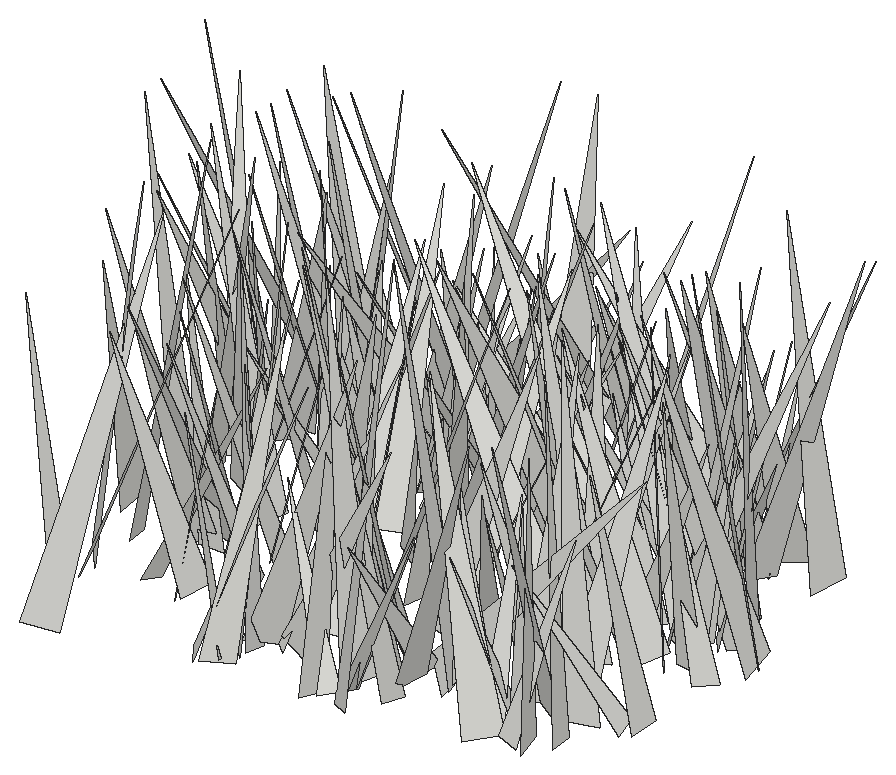
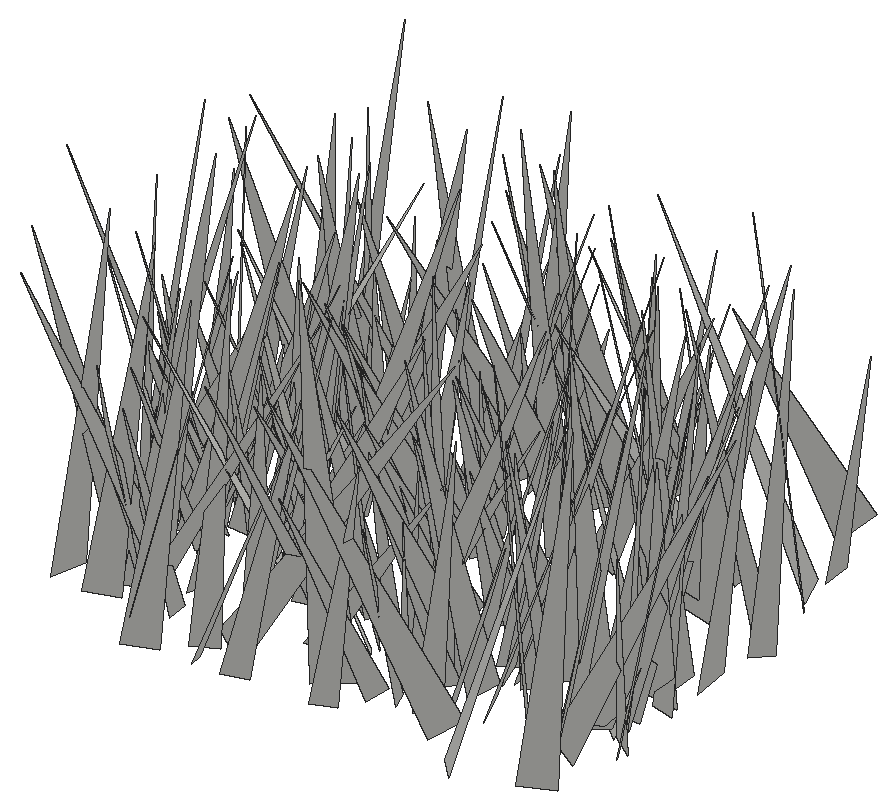
# SketchUp Ruby script. Lengths in inches.
U = 1.inch
M = Sketchup.active_model
def pt(a) = Geom::Point3d.new(a.map { |v| v * U })
def face(e, loops, mat)
  f = e.add_face(loops[0].map { |a| pt(a) })
  loops[1..].each { |l| e.add_face(l.map { |a| pt(a) }).erase! }
  f.material = f.back_material = mat if mat
  f
end
# faces: each face lists its corners as indices into pts; further lists are holes
def faces(e, pts, list, mat = nil) = list.each { |f| face(e, (f[0].is_a?(Array) ? f : [f]).map { |l| l.map { |i| pts[i] } }, mat) }
# xy, xz, yz: faces in a plane at the given z, y or x. An outline is a flat list of corners, or four numbers for a rectangle; further outlines are holes
def ring(l) = l.size == 4 ? [[l[0], l[1]], [l[2], l[1]], [l[2], l[3]], [l[0], l[3]]] : l.each_slice(2).to_a
def flat(e, list, mat, &to3) = list.each { |f| face(e, (f[0].is_a?(Array) ? f : [f]).map { |l| ring(l).map { |u, v| to3.(u, v) } }, mat) }
def xy(e, z, list, mat = nil) = flat(e, list, mat) { |x, y| [x, y, z] }
def xz(e, y, list, mat = nil) = flat(e, list, mat) { |x, z| [x, y, z] }
def yz(e, x, list, mat = nil) = flat(e, list, mat) { |y, z| [x, y, z] }
def lines(e, pts, list) = list.each { |a, b| e.add_line(pt(pts[a]), pt(pts[b])) }
# prism: a flat outline (further loops are holes) pulled along v
def prism(e, loops, v, mat = nil)
  f = face(e, loops, mat); d = Geom::Vector3d.new(v.map { |x| x * U })
  f.pushpull(f.normal.samedirection?(d) ? d.length : -d.length)
end
def box(e, o, s, mat = nil) = prism(e, [[o, [o[0] + s[0], o[1], o[2]], [o[0] + s[0], o[1] + s[1], o[2]], [o[0], o[1] + s[1], o[2]]]], [0, 0, s[2]], mat)
def at(x, y, z, deg = 0) = Geom::Transformation.translation(pt([x, y, z])) * Geom::Transformation.rotation(ORIGIN, Z_AXIS, deg.degrees)
def axes(o, x, y, z) = Geom::Transformation.new([*x, 0, *y, 0, *z, 0, *pt(o).to_a, 1])
def part(name) = M.definitions.add(name)
# library, detail: a bought-in or finely detailed component or shape, given as its bounding box
def library(name, o, s) = part(name).tap { |d| box(d.entities, o, s) }
def detail(e, o, s) = box(e.add_group.entities, o, s)
def put(e, d, t, mat = nil) = e.add_instance(d, t).tap { |i| i.material = mat if mat }
def group(e, t, mat = nil) = e.add_group.tap { |g| g.transformation = t; g.material = mat if mat }.entities
root = M.entities
c1 = part("fur_instance\#9")
p = [[0.8125,0,1.79],[0.67,-0.02,1.48],[0,-0.11,0],[0,0.11,0]]
faces(c1.entities,p,[[0,1,2,3]])
put(root,c1,axes([79.35,396.46,-27.1],[3.86855,-0.79855,0.19754],[-0.81455,-3.85123,0.38332],[-0.11496,0.41562,3.93147]))
put(root,c1,axes([73.47,395.12,-27.1],[4.56753,3.50086,0.36537],[3.49009,-4.58212,0.27435],[-0.45689,-0.00383,5.74831]))
put(root,c1,axes([78.98,395.87,-27.1],[-2.26305,3.25436,0.20739],[3.19812,2.16563,0.91504],[-0.63708,-0.68879,3.8568]))
put(root,c1,axes([74.48,395.55,-27.1],[-4.28089,-1.18354,0.47624],[-1.27514,3.91753,-1.72642],[-0.03977,1.79046,4.09221]))
put(root,c1,axes([86.23,399.45,-27.1],[-2.59583,-7.17613,0.91864],[-6.91744,2.74775,1.9178],[2.11891,0.17907,7.38629]))
put(root,c1,axes([66.48,396.31,-27.1],[-5.31115,0.249,1.00047],[0.14264,5.37711,-0.58108],[1.02108,0.54405,5.28514]))
put(root,c1,axes([76,397.62,-27.1],[0.54416,-5.67013,1.84078],[-5.27926,0.40028,2.79359],[2.76917,1.87733,4.9641]))
put(root,c1,axes([80.71,398.32,-27.1],[6.6655,-1.52718,0.22941],[-1.49066,-6.62814,-0.81212],[-0.40351,-0.74118,6.78982]))
put(root,c1,axes([80.7,399.42,-27.1],[3.27584,-2.78093,0.2499],[-2.38988,-2.99185,-1.96583],[-1.44378,-1.35736,3.82103]))
put(root,c1,axes([86.86,397.32,-27.1],[5.38301,1.51294,2.42188],[1.75431,-5.82988,-0.25732],[-2.2532,-0.92457,5.58566]))
put(root,c1,axes([74.49,395.2,-27.1],[-4.85985,3.92503,1.53679],[3.59209,5.08366,-1.6245],[2.20555,0.36911,6.032]))
put(root,c1,axes([85.26,396.76,-27.1],[-5.2406,4.407,1.34408],[4.57378,5.22157,0.71269],[0.55566,-1.41624,6.81011]))
put(root,c1,axes([78.59,395.48,-27.1],[-7.01527,0.64484,2.20419],[0.06996,7.14138,-1.86657],[2.29551,1.75305,6.79307]))
put(root,c1,axes([68.03,393.23,-27.1],[-6.65412,4.03174,0.74119],[3.28122,6.08544,-3.64454],[2.45722,2.79179,6.87384]))
put(root,c1,axes([74.87,397.32,-27.1],[5.22316,-4.20753,1.34718],[-4.41725,-5.01042,1.47756],[-0.07792,1.998,6.54228]))
put(root,c1,axes([79.34,397.22,-27.1],[-7.46216,1.5868,2.36089],[1.65538,7.81249,-0.01867],[2.31332,-0.47194,7.62898]))
put(root,c1,axes([70.68,398.75,-27.1],[-5.0365,1.95588,2.0654],[2.56555,4.93734,1.5806],[1.22852,-2.29236,5.16658]))
put(root,c1,axes([85.71,398.26,-27.1],[-3.47043,-1.20582,0.35373],[-1.16309,3.47557,0.43669],[0.47575,-0.29913,3.64791]))
put(root,c1,axes([70.1,398.38,-27.1],[4.41125,2.39111,1.26664],[2.67652,-4.21168,-1.37073],[-0.39751,-1.82353,4.82677]))
put(root,c1,axes([86.12,397.06,-27.1],[1.17442,4.10835,0.87727],[4.16659,-1.02282,-0.78793],[0.5364,-1.0501,4.19964]))
put(root,c1,axes([79.95,395.3,-27.1],[4.59054,6.55576,1.84003],[6.00661,-4.94402,2.62946],[-3.20693,0.124,7.5589]))
put(root,c1,axes([79.47,399.59,-27.1],[-3.91198,-5.41617,1.52932],[-5.50053,4.07361,0.35664],[1.19076,1.02376,6.67167]))
put(root,c1,axes([74.93,396.75,-27.1],[-6.75602,-0.97126,1.58692],[-1.43223,6.52998,-2.10085],[1.1876,2.34979,6.49412]))
put(root,c1,axes([85.06,397.44,-27.1],[-1.60634,4.05647,0.77587],[4.09581,1.67158,-0.25963],[0.53033,-0.623,4.35521]))
put(root,c1,axes([74.64,396.21,-27.1],[5.18637,5.57386,2.23152],[5.04396,-5.64447,2.37581],[-3.2567,0.13438,7.23339]))
put(root,c1,axes([81.04,396.94,-27.1],[-7.866,-1.33504,0.19154],[-1.32695,7.45779,-2.51268],[-0.24134,2.50839,7.5725]))
put(root,c1,axes([83.48,398.91,-27.1],[-3.08367,2.72536,1.78242],[3.08151,3.23588,0.38343],[1.05304,-1.48834,4.09751]))
put(root,c1,axes([72.75,399.54,-27.1],[-2.53313,-4.37285,1.78451],[-4.47538,2.86942,0.67851],[1.50904,1.16947,5.00781]))
put(root,c1,axes([66.24,398.49,-27.1],[5.70767,4.90783,2.44546],[5.23724,-5.92496,-0.33273],[-1.62433,-1.85811,7.52021]))
put(root,c1,axes([66.44,397.78,-27.1],[7.55875,3.30018,0.58934],[3.3113,-7.57673,-0.04195],[-0.52327,-0.27436,8.24768]))
put(root,c1,axes([81.13,399.31,-27.1],[5.03462,6.0848,0.40692],[5.07887,-3.8915,-4.64748],[3.37572,-3.22012,6.38538]))
put(root,c1,axes([85.7,398.17,-27.1],[-3.90689,0.46662,1.17538],[0.26281,4.03296,-0.72751],[1.23701,0.61693,3.86682]))
put(root,c1,axes([88.72,400.48,-27.1],[-4.09373,-0.36711,0.23804],[-0.24891,3.79616,1.57392],[0.35983,-1.55061,3.79686]))
put(root,c1,axes([75.23,397.73,-27.1],[3.93505,4.96293,0.50565],[4.97977,-3.8695,-0.7745],[0.29702,-0.87596,6.28613]))
put(root,c1,axes([72.21,400.37,-27.1],[-5.06877,-1.96642,0.89661],[-1.81084,5.11214,0.97466],[1.17965,-0.60192,5.34876]))
put(root,c1,axes([87.65,398.17,-27.1],[-6.31895,-1.30533,1.91515],[-1.71826,6.37081,-1.32708],[1.5554,1.73484,6.31441]))
put(root,c1,axes([81.94,399.49,-27.1],[-7.67624,-2.38765,2.18106],[-2.53698,7.93,-0.24775],[2.0054,0.89261,8.03519]))
put(root,c1,axes([70.76,401.5,-27.1],[-3.28751,-5.48957,1.02333],[-5.33666,3.43821,1.29963],[1.64396,0.18343,6.2653]))
put(root,c1,axes([68.89,398.44,-27.1],[4.92318,-0.35306,0.35659],[-0.43613,-4.74982,1.31852],[-0.24819,1.34315,4.75646]))
put(root,c1,axes([78.87,397.71,-27.1],[-4.6642,0.46344,0.8289],[0.1067,4.38406,-1.85075],[0.94364,1.79496,4.30631]))
put(root,c1,axes([69.5625,402.18,-27.1],[-1.29873,-6.18935,0.13887],[-6.18983,1.30082,0.08883],[0.11547,0.11765,6.32352]))
put(root,c1,axes([74.83,401.34,-27.1],[0.15208,-7.64456,1.76209],[-7.47072,0.39677,2.36609],[2.3943,1.72356,7.27077]))
put(root,c1,axes([84.03,400.91,-27.1],[-0.63245,-3.70623,0.66325],[-3.76509,0.62047,-0.12308],[-0.01169,0.67448,3.75779]))
put(root,c1,axes([89.28,400.84,-27.1],[-5.12264,0.34016,1.65759],[0.60899,5.30124,0.79415],[1.57874,-0.94118,5.07212]))
put(root,c1,axes([79.77,398.69,-27.1],[-7.1733,-2.93015,0.73361],[-2.97558,6.52972,-3.01478],[-0.51951,3.05896,7.13815]))
put(root,c1,axes([68.76,401.6,-27.1],[-0.74223,-7.02206,1.66779],[-7.14663,0.48084,-1.156],[-1.00829,1.76103,6.96591]))
put(root,c1,axes([77.93,401.3125,-27.1],[-1.24841,-4.57565,0.91997],[-4.66472,1.19209,-0.401],[-0.15278,0.99186,4.72592]))
put(root,c1,axes([80.73,402.82,-27.1],[5.43533,-0.93824,0.08866],[-0.80913,-4.91198,-2.3767],[-0.48317,-2.32876,4.97739]))
put(root,c1,axes([64.89,402.51,-27.1],[6.40589,-1.32849,1.4611],[-0.83624,-6.31798,-2.07823],[-1.78897,-1.80373,6.20333]))
put(root,c1,axes([87.33,399.73,-27.1],[-0.74799,6.94474,2.29097],[7.27165,0.46217,0.97314],[-0.77532,-2.36525,6.91678]))
put(root,c1,axes([73.6,400.71,-27.1],[-0.2537,5.53184,2.90433],[5.7111,-0.97344,2.35297],[-2.53371,-2.74807,5.0129]))
put(root,c1,axes([79.5,396.64,-27.1],[6.78257,3.66457,1.14232],[2.83952,-6.35069,3.51329],[-2.58286,2.6414,6.86216]))
put(root,c1,axes([72.43,397.28,-27.1],[5.32818,4.49942,0.50618],[3.89144,-4.95023,3.04014],[-2.31467,2.03493,6.2763]))
put(root,c1,axes([70.41,400.74,-27.1],[4.87544,3.99495,1.42226],[4.19795,-4.85335,-0.75795],[-0.59966,-1.4959,6.2574]))
put(root,c1,axes([84.94,399.91,-27.1],[-5.03968,3.97301,2.20808],[3.85689,5.48236,-1.06156],[2.40517,-0.46656,6.329]))
put(root,c1,axes([69.17,401.48,-27.1],[-0.51846,-5.08764,2.15235],[-5.51728,0.36879,-0.45728],[-0.27624,2.18298,5.0935]))
put(root,c1,axes([86.57,400.06,-27.1],[-2.09917,6.50868,2.06271],[6.47308,2.58358,-1.56477],[2.17184,-1.40938,6.65739]))
put(root,c1,axes([74.07,402.51,-27.1],[-6.35383,-3.10693,1.06991],[-3.1587,6.41685,-0.12448],[0.9057,0.58302,7.07168]))
put(root,c1,axes([80.125,402.47,-27.1],[-0.83956,4.61048,2.28414],[5.1209,0.52371,0.82514],[-0.50027,-2.37653,4.61309]))
put(root,c1,axes([79.14,401.81,-27.1],[2.35297,-5.60644,2.50548],[-6.03434,-1.6135,2.05656],[1.13856,3.03489,5.72182]))
put(root,c1,axes([77.17,403.02,-27.1],[4.35751,-1.25814,0.68683],[-1.21703,-4.4086,-0.35441],[-0.75729,-0.15444,4.52164]))
put(root,c1,axes([82.36,403.53,-27.1],[-3.76395,0.54517,1.33918],[0.93594,3.7652,1.09781],[1.1021,-1.33566,3.64133]))
put(root,c1,axes([66.54,400.58,-27.1],[6.51752,3.06728,2.32468],[2.5593,-6.86862,1.88745],[-2.87443,0.8392,6.95153]))
put(root,c1,axes([71.23,402.34,-27.1],[3.50621,1.98379,0.78234],[2.0421,-3.55715,-0.13217],[-0.61424,-0.50223,4.02634]))
put(root,c1,axes([76.26,399.25,-27.1],[-5.16112,5.15909,0.10388],[4.87926,4.92701,-2.27629],[1.67923,1.54029,6.93338]))
put(root,c1,axes([73.25,405.4,-27.1],[-4.74866,-3.13825,0.27488],[-2.86364,4.50737,1.98925],[1.31291,-1.51952,5.33303]))
put(root,c1,axes([87.54,402.89,-27.1],[-7.14593,-4.06809,0.00282],[-3.91681,6.87864,-2.22635],[-1.09909,1.93614,7.91562]))
put(root,c1,axes([79.96,401.41,-27.1],[4.40688,2.08061,0.00975],[2.02682,-4.29803,1.08102],[-0.47012,0.97349,4.75194]))
put(root,c1,axes([67.52,405.37,-27.1],[-1.15928,-6.64992,1.1524],[-6.36185,1.46707,2.06591],[2.25307,0.72087,6.42631]))
put(root,c1,axes([84.09,403.76,-27.1],[-6.8866,-1.44069,2.04712],[-1.4724,7.17733,0.09795],[2.02444,0.3193,7.035]))
put(root,c1,axes([84.875,403.37,-27.1],[-1.73257,6.85044,2.42635],[7.20837,1.30251,1.46979],[-0.92468,-2.68187,6.91158]))
put(root,c1,axes([82.83,402.4375,-27.1],[5.42276,2.60915,0.23648],[2.58182,-5.41452,0.53583],[-0.44475,0.3811,5.9939]))
put(root,c1,axes([73,404.14,-27.1],[-5.77727,-4.35757,2.82703],[-4.73437,6.15702,-0.18467],[2.13687,1.8601,7.23403]))
put(root,c1,axes([74.89,405.39,-27.1],[-1.05562,-3.90874,0.84941],[-3.49411,1.32871,1.77194],[1.94702,0.26528,3.64044]))
put(root,c1,axes([83.32,403.73,-27.1],[-5.71693,5.39586,0.3581],[5.20349,5.34707,2.50186],[-1.47216,-2.05434,7.45247]))
put(root,c1,axes([87.9375,405.17,-27.1],[-0.39451,-5.89979,1.57703],[-6.09619,0.47415,0.24879],[0.36204,1.55494,5.90773]))
put(root,c1,axes([86.67,405.16,-27.1],[-4.90081,-4.60842,2.76686],[-4.75517,5.4628,0.67611],[2.50627,1.35324,6.69315]))
put(root,c1,axes([89.03,404.62,-27.1],[-2.03282,4.17049,1.29504],[4.34211,1.77825,1.08919],[-0.46493,-1.62705,4.50988]))
put(root,c1,axes([86.41,404.92,-27.1],[-6.01632,2.22797,0.81671],[2.32649,5.97644,0.83455],[0.46722,-1.07014,6.36109]))
put(root,c1,axes([68.51,404.1,-27.1],[-3.5127,-1.06556,1.8883],[-1.54789,3.74984,-0.76344],[1.51826,1.35772,3.59049]))
put(root,c1,axes([74.625,403.36,-27.1],[3.7445,3.22853,1.26331],[2.91821,-3.9391,1.41711],[-1.87174,0.31742,4.73672]))
put(root,c1,axes([69.54,404.39,-27.1],[-7.31689,1.04904,1.18508],[0.99417,7.40794,-0.41938],[1.23147,0.25252,7.3798]))
put(root,c1,axes([78.73,402.34,-27.1],[5.48783,2.36239,1.1528],[1.72376,-5.24883,2.55038],[-1.98455,1.97355,5.40302]))
put(root,c1,axes([89.56,406.93,-27.1],[-7.48109,-1.28394,1.71532],[-0.94889,7.57103,1.5286],[1.92105,-1.26035,7.43496]))
put(root,c1,axes([65.84,405.77,-27.1],[6.8953,0.9557,1.85973],[1.13553,-7.09282,-0.56526],[-1.75571,-0.83402,6.93822]))
put(root,c1,axes([65.09,405.14,-27.1],[-7.05246,-0.20222,1.59365],[-0.38202,7.18084,-0.77939],[1.56034,0.84409,7.01218]))
put(root,c1,axes([83.24,405.64,-27.1],[3.99343,-3.31881,2.86458],[-3.84361,-4.5142,0.12826],[-2.10878,1.94301,5.19091]))
put(root,c1,axes([79.55,409.56,-27.1],[6.1806,-4.85252,1.92283],[-3.89661,-6.27237,-3.30423],[-3.47285,-1.59827,7.12944]))
put(root,c1,axes([65.15,407.8125,-27.1],[-2.48382,-6.27006,1.58629],[-6.2632,2.75568,1.08533],[1.61318,1.04494,6.65621]))
put(root,c1,axes([78.77,403.73,-27.1],[-3.2571,5.60614,0.8435],[5.30317,3.35677,-1.83235],[2.00417,0.22864,6.21933]))
put(root,c1,axes([89.16,407.24,-27.1],[-5.20637,-5.83633,2.28098],[-6.06397,5.44004,0.07832],[1.57922,1.64775,7.82067]))
put(root,c1,axes([72.2,404.8,-27.1],[5.46763,0.70402,1.09334],[0.38726,-5.3924,1.5356],[-1.2414,1.41859,5.29457]))
put(root,c1,axes([66.1,408.98,-27.1],[2.22572,-6.24997,0.53761],[-6.03536,-2.28904,-1.62473],[-1.71046,-0.05581,6.43243]))
put(root,c1,axes([87.14,406.23,-27.1],[3.46953,-2.67132,1.40146],[-2.94376,-3.4648,0.68347],[-0.65905,1.41311,4.3251]))
put(root,c1,axes([84.59,406.27,-27.1],[3.70527,-2.55389,0.75103],[-2.66189,-3.54115,1.0909],[0.02774,1.32414,4.36593]))
put(root,c1,axes([66.91,407.51,-27.1],[4.97052,1.68586,2.30908],[2.28367,-5.12743,-1.17229],[-1.72012,-1.9358,5.11604]))
put(root,c1,axes([83.84,404.37,-27.1],[2.91229,5.1803,0.24137],[5.15397,-2.92189,0.52374],[-0.57474,0.04729,5.91968]))
put(root,c1,axes([82.65,408.57,-27.1],[5.01646,-0.03484,2.02413],[0.79085,-4.94522,-2.0451],[-1.86357,-2.19241,4.58078]))
put(root,c1,axes([78.0625,403.32,-27.1],[7.02675,2.35333,1.41841],[1.60681,-6.67867,3.12071],[-2.22895,2.60433,6.72121]))
put(root,c1,axes([70.99,405.51,-27.1],[0.97276,4.45119,0.9772],[4.35496,-1.20232,1.14148],[-1.3425,-0.67498,4.41093]))
put(root,c1,axes([69.21,408.3125,-27.1],[4.90376,-2.85552,0.72078],[-2.73926,-4.93651,-0.92072],[-1.08166,-0.44414,5.59939]))
put(root,c1,axes([74.5625,408.62,-27.1],[6.47505,-0.26988,1.20187],[0.07267,-6.33614,-1.81428],[-1.22965,-1.79557,6.22153]))
put(root,c1,axes([85.27,408.7,-27.1],[-5.50457,-1.9976,0.13924],[-1.94432,5.42927,1.02602],[0.47897,-0.91798,5.76524]))
put(root,c1,axes([84.88,407,-27.1],[0.57769,-3.84784,2.16026],[-4.16363,-1.197,-1.01866],[-1.46176,1.88882,3.75525]))
put(root,c1,axes([86.97,406.97,-27.1],[3.29573,-2.04708,1.27302],[-2.29025,-3.33183,0.57152],[-0.75223,1.17531,3.83742]))
put(root,c1,axes([71.38,408.64,-27.1],[3.60801,-2.69307,1.35493],[-2.4926,-3.85347,-1.02171],[-1.69571,-0.06573,4.3848]))
put(root,c1,axes([80.42,407.67,-27.1],[6.04949,2.12455,0.78775],[2.22415,-5.99674,-0.90711],[-0.43293,-1.1207,6.34722]))
put(root,c1,axes([88.34,407.46,-27.1],[-1.48445,-5.73193,2.26963],[-5.6541,0.33538,-2.85107],[-2.45713,2.69116,5.18942]))
put(root,c1,axes([65.57,410.18,-27.1],[-4.43936,-4.76816,0.23664],[-4.66276,4.39992,1.18262],[1.02469,-0.63608,6.40661]))
put(root,c1,axes([80.88,407.76,-27.1],[4.18181,1.0835,0.53294],[1.13424,-4.18373,-0.39425],[-0.41412,-0.51766,4.30187]))
put(root,c1,axes([70.5,408.8,-27.1],[-7.46338,-1.41905,1.28497],[-1.31215,7.55774,0.72509],[1.39396,-0.48353,7.56241]))
put(root,c1,axes([86.04,407.79,-27.1],[-6.89397,4.20656,1.53795],[4.42912,6.82252,1.19307],[0.66584,-1.82904,7.9874]))
put(root,c1,axes([84.45,409.55,-27.1],[-3.67064,-4.64361,1.03864],[-4.58105,3.8034,0.81465],[1.28682,0.29416,5.86285]))
put(root,c1,axes([70.83,412.82,-27.1],[-6.33754,-5.19611,0.8236],[-4.02771,5.62162,4.47406],[3.3846,-3.03975,6.86635]))
put(root,c1,axes([88.79,407.67,-27.1],[-6.27895,-2.5321,2.5957],[-2.9165,6.61067,-0.60625],[2.15482,1.56906,6.74309]))
put(root,c1,axes([67.01,410.76,-27.1],[-3.15588,-6.30761,0.73503],[-6.08642,3.23856,1.65924],[1.81157,-0.10755,6.85511]))
put(root,c1,axes([77.24,408.6875,-27.1],[3.19208,-3.97574,0.46961],[-3.91795,-2.97897,1.41133],[0.82265,1.2392,4.89939]))
put(root,c1,axes([85.54,407.4,-27.1],[3.97232,6.71602,1.21655],[6.692,-3.55551,-2.22255],[1.34242,-2.14887,7.47961]))
put(root,c1,axes([72.18,406.99,-27.1],[-2.71251,3.20119,0.88639],[3.03008,2.85354,-1.03292],[1.36084,0.02704,4.06674]))
put(root,c1,axes([66.04,410.14,-27.1],[2.61473,-6.42495,0.46001],[-6.33227,-2.47287,1.45453],[1.18065,0.96609,6.78241]))
put(root,c1,axes([86.2,406.02,-27.1],[3.78632,3.0497,0.88341],[2.42458,-3.66486,2.25998],[-2.05,1.29824,4.30457]))
put(root,c1,axes([73.32,406.37,-27.1],[-3.56616,5.34471,0.77163],[5.27091,3.64619,-0.89538],[1.17426,-0.13507,6.36253]))
put(root,c1,axes([82.24,409.24,-27.1],[-2.77092,-3.22119,0.17285],[-3.17409,2.68192,-0.90354],[-0.57541,0.71776,4.15182]))
put(root,c1,axes([86.47,406.26,-27.1],[3.93079,5.90323,1.06815],[5.73682,-4.07234,1.39466],[-1.7544,-0.09002,6.95371]))
put(root,c1,axes([87.5,407.2,-27.1],[-3.93965,-2.75758,3.63418],[-3.8658,4.56754,-0.72493],[2.42222,2.80458,4.7539]))
put(root,c1,axes([75.03,408.52,-27.1],[6.15775,0.09619,0.89999],[0.03195,-6.20791,0.44493],[-0.90455,0.43558,6.14241]))
put(root,c1,axes([65.3,409.69,-27.1],[-2.6203,-2.567,1.06702],[-2.53846,2.80716,0.51965],[1.13325,0.35259,3.63117]))
put(root,c1,axes([80.96,409.45,-27.1],[-0.62514,-3.66803,1.11265],[-3.82799,0.53943,-0.37244],[-0.19721,1.15663,3.70223]))
put(root,c1,axes([74.94,410.63,-27.1],[-1.76635,-5.02439,0.02248],[-4.81779,1.68692,-1.51928],[-1.42615,0.52421,5.10454]))
put(root,c1,axes([71.01,409.14,-27.1],[-6.09908,-2.25868,1.59557],[-2.41433,6.23322,-0.4051],[1.3485,0.94419,6.49124]))
put(root,c1,axes([65.8,409.87,-27.1],[-4.26864,3.3889,1.68719],[3.78174,3.93314,1.66776],[0.17248,-2.36607,5.18889]))
put(root,c1,axes([69.72,409.3125,-27.1],[2.82184,-3.33686,1.43593],[-3.57868,-2.86589,0.37288],[-0.62414,1.34588,4.35412]))
put(root,c1,axes([65.79,407.24,-27.1],[-1.06159,6.87885,0.56166],[6.76624,0.92524,1.45707],[-1.36093,-0.76575,6.80607]))
put(root,c1,axes([82.52,408.76,-27.1],[0.52075,4.40411,1.27547],[4.58416,-0.47433,-0.2338],[0.09203,-1.29345,4.42863]))
put(root,c1,axes([84.99,412.25,-27.1],[5.51708,-5.76072,0.82028],[-5.55442,-5.55067,-1.6234],[-1.73412,-0.54876,7.80952]))
put(root,c1,axes([74.58,406.69,-27.1],[5.42,0.95377,1.93695],[-0.10115,-5.11614,2.80228],[-2.15667,2.63692,4.73638]))
put(root,c1,axes([83.53,411.18,-27.1],[-6.08575,-1.31512,1.93305],[-0.80976,6.24223,1.69745],[2.19329,-1.34444,5.99037]))
put(root,c1,axes([73.6875,408.32,-27.1],[-0.65991,4.20046,0.70673],[4.09857,0.8209,-1.05196],[1.15975,-0.51096,4.1198]))
put(root,c1,axes([73.64,409.54,-27.1],[-2.04646,-5.42862,2.85461],[-5.95901,2.47232,0.42963],[1.45222,2.49488,5.78561]))
put(root,c1,axes([72.125,409.73,-27.1],[-3.54918,2.04608,0.76374],[2.14815,3.53344,0.51649],[0.39398,-0.83357,4.06404]))
put(root,c1,axes([80.89,409.34,-27.1],[-4.85114,5.94494,0.47809],[5.69058,4.42924,2.66526],[-1.78556,-2.03568,7.19529]))
put(root,c1,axes([74.8125,410.74,-27.1],[5.2345,0.58731,0.96902],[0.7581,-5.21929,-0.93179],[-0.84215,-1.04786,5.18428]))
put(root,c1,axes([87.11,409.85,-27.1],[-3.42512,-4.29344,1.99666],[-4.721,3.28594,-1.03273],[0.36395,2.21827,5.39431]))
put(root,c1,axes([74.28,410.77,-27.1],[1.30343,6.50873,4.51627],[7.0846,-3.00591,2.28737],[-3.54523,-3.61388,6.23141]))
put(root,c1,axes([74.25,410.78,-27.1],[-3.40135,-0.48301,1.73948],[-0.24917,3.80046,0.56808],[1.78802,-0.38922,3.38818]))
put(root,c1,axes([72.37,409.8,-27.1],[4.7492,-0.22527,1.39473],[-0.44396,-4.88167,0.72329],[-1.34124,0.81823,4.6992]))
put(root,c1,axes([84.89,409.09,-27.1],[0.96438,4.41888,0.40988],[4.43511,-0.94495,-0.24768],[0.15571,-0.45288,4.5161]))
put(root,c1,axes([64.78,410.67,-27.1],[-6.58446,-3.61184,1.85584],[-3.84727,6.67992,-0.64953],[1.29924,1.4758,7.48189]))
put(root,c1,axes([66.12,412.28,-27.1],[-2.71774,-6.73125,0.47193],[-6.54696,2.5072,-1.9416],[-1.63394,1.15011,6.99472]))
put(root,c1,axes([78.18,407.99,-27.1],[5.42222,1.22065,1.50489],[0.3801,-5.05507,2.73075],[-1.90005,2.47215,4.84081]))
put(root,c1,axes([75.9,410.875,-27.1],[3.62695,2.69385,0.06353],[2.59465,-3.4627,-1.30122],[0.7271,-1.08099,4.32648]))
put(root,c1,axes([69.95,411.56,-27.1],[-6.57116,-2.81105,0.67584],[-2.85659,6.57143,-0.44162],[0.44572,0.67315,7.13352]))
put(root,c1,axes([70.97,410.625,-27.1],[6.40804,-1.16691,1.44574],[-1.35043,-6.49108,0.74636],[-1.27601,1.00946,6.47052]))
put(root,c1,axes([66.57,411.87,-27.1],[-5.55068,-3.03255,1.58004],[-3.06213,5.7489,0.27653],[1.52193,0.50669,6.31901]))
put(root,c1,axes([67.4375,410.99,-27.1],[1.6675,5.06938,1.93589],[5.41393,-1.41673,-0.95346],[0.36831,-2.12629,5.25072]))
put(root,c1,axes([76.36,409.97,-27.1],[3.82909,4.88275,1.88302],[4.81565,-4.20088,1.10051],[-2.04855,-0.74856,6.10673]))
put(root,c1,axes([77.625,411.79,-27.1],[-3.75948,2.94392,0.27379],[2.73653,3.29698,2.12525],[-1.1194,-1.82718,4.27594]))
put(root,c1,axes([85.93,413.58,-27.1],[3.11864,-5.68803,0.55795],[-5.6529,-3.16353,-0.65398],[-0.84244,0.17118,6.45383]))
put(root,c1,axes([72.13,411.02,-27.1],[0.15011,3.96157,1.30257],[3.86973,0.35348,-1.52101],[1.55431,-1.26265,3.66102]))
put(root,c1,axes([64.6875,410.66,-27.1],[1.72426,4.07776,1.35625],[4.04188,-2.03524,0.98061],[-1.4597,-0.81871,4.31736]))
put(root,c1,axes([84.28,413.9,-27.1],[-5.52668,-3.91053,1.22579],[-3.5737,5.60606,1.77193],[2.00587,-0.78663,6.53427]))
put(root,c1,axes([80.7,414.28,-27.1],[0.16634,-6.6201,0.01552],[-6.42128,-0.15757,1.61124],[1.61035,0.05552,6.42319]))
put(root,c1,axes([71.54,413.1,-27.1],[3.51488,-3.51732,0.75482],[-3.443,-3.59499,-0.71937],[-1.04262,0.01399,4.9202]))
put(root,c1,axes([84.29,413.4,-27.1],[-7.00038,0.48524,0.02911],[0.47648,6.76613,1.79834],[-0.09628,-1.796,6.78283]))
put(root,c1,axes([79.54,413.08,-27.1],[-6.2182,-2.45212,1.53392],[-2.39925,6.40419,0.51167],[1.61537,0.0727,6.66461]))
put(root,c1,axes([81.72,408.29,-27.1],[5.15692,6.28398,0.1894],[5.87834,-4.90651,2.73667],[-2.22922,1.59869,7.6546]))
put(root,c1,axes([85.41,412.33,-27.1],[1.48907,3.83094,1.46531],[4.09712,-1.31638,-0.722],[0.19182,-1.62223,4.04625]))
put(root,c1,axes([74.06,411.18,-27.1],[1.76698,3.75792,1.11012],[3.4505,-2.06932,1.51278],[-1.85698,-0.26926,3.86726]))
put(root,c1,axes([80.43,411.66,-27.1],[-5.1029,2.41175,1.4356],[2.37658,5.2976,-0.4521],[1.4931,-0.1897,5.62599]))
put(root,c1,axes([85.68,411.8125,-27.1],[6.84778,-1.68967,1.39359],[-1.92956,-6.81846,1.21431],[-1.03628,1.53061,6.94784]))
put(root,c1,axes([66.49,413.55,-27.1],[5.45903,4.38742,2.52703],[5.0114,-5.21201,-1.77686],[-0.72192,-3.00365,6.77446]))
put(root,c1,axes([79.92,413.79,-27.1],[-3.41379,-7.32141,0.63154],[-6.65452,2.7845,-3.69049],[-3.11756,2.07349,7.18591]))
put(root,c1,axes([87.94,412.9375,-27.1],[-7.15931,0.95304,2.49675],[1.12982,7.54938,0.35801],[2.42189,-0.70454,7.21359]))
put(root,c1,axes([84.82,411.14,-27.1],[6.67299,1.88656,0.54903],[1.75109,-6.59185,1.3677],[-0.89119,1.17381,6.79833]))
put(root,c1,axes([72.63,409.39,-27.1],[-6.96158,0.42843,3.50828],[-1.43896,6.73486,-3.67782],[3.22816,3.92599,5.92628]))
put(root,c1,axes([83.04,412.9,-27.1],[4.10361,0.18993,0.89205],[0.09258,-4.17709,0.46346],[-0.90734,0.43277,4.08178]))
put(root,c1,axes([78.53,415.28,-27.1],[3.73723,-3.51523,0.8829],[-3.22394,-3.80362,-1.49732],[-1.65607,-0.52811,4.90732]))
put(root,c1,axes([76.29,411.71,-27.1],[1.18506,6.07091,0.5983],[5.8889,-0.9794,-1.72625],[1.5921,-0.89616,5.93973]))
put(root,c1,axes([75.49,413.43,-27.1],[-3.47226,6.33449,3.63746],[6.89094,4.17667,-0.69553],[2.42317,-2.80055,7.19017]))
put(root,c1,axes([72.92,412.99,-27.1],[3.22488,1.438,0.95498],[1.40641,-3.36208,0.31327],[-1.00092,-0.09099,3.51704]))
put(root,c1,axes([82.5,415.7,-27.1],[3.11347,-5.57932,0.56956],[-5.54553,-3.1599,-0.63956],[-0.83685,0.18197,6.35716]))
put(root,c1,axes([80.36,415.22,-27.1],[-4.41173,-1.92667,0.46008],[-1.77307,4.34177,1.17998],[0.88316,-0.90777,4.66723]))
put(root,c1,axes([70.28,413.61,-27.1],[4.62991,-4.98565,0.093],[-4.3743,-3.99984,3.34189],[2.39393,2.33366,5.92659]))
put(root,c1,axes([65.17,414.89,-27.1],[3.62749,-5.55241,1.8821],[-5.65778,-3.89547,-0.58748],[-1.5366,1.23544,6.60627]))
put(root,c1,axes([68.53,415.79,-27.1],[-4.85913,-4.7221,0.69622],[-4.68141,4.90862,0.61965],[0.93132,0.03646,6.74725]))
put(root,c1,axes([73.76,413.18,-27.1],[3.57113,-2.0967,0.79041],[-2.23153,-3.1932,1.61171],[0.20288,1.78359,3.81464]))
put(root,c1,axes([74.77,414.97,-27.1],[2.46831,-3.73303,1.12427],[-3.72872,-2.64901,-0.60947],[-1.13849,0.58247,4.43358]))
